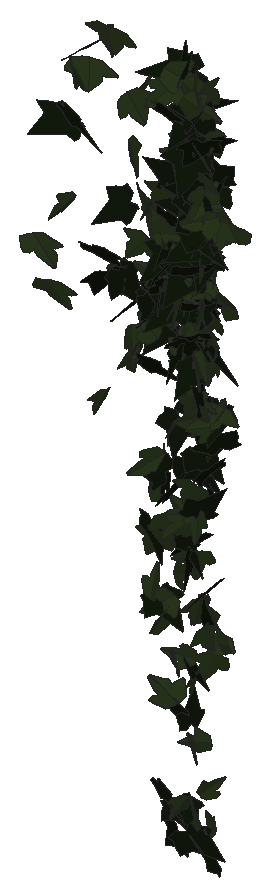
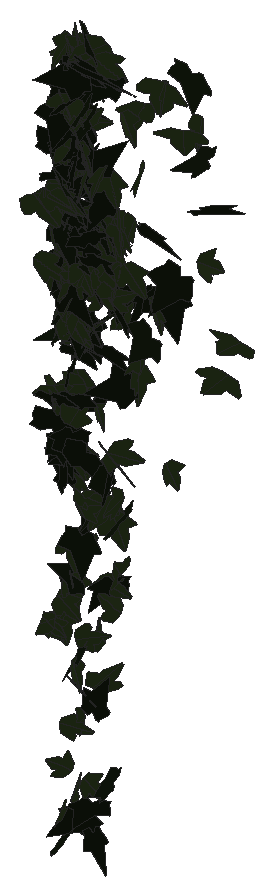
# SketchUp Ruby script. Lengths in millimetres.
U = 1.mm
M = Sketchup.active_model
def pt(a) = Geom::Point3d.new(a.map { |v| v * U })
def face(e, loops, mat)
  f = e.add_face(loops[0].map { |a| pt(a) })
  loops[1..].each { |l| e.add_face(l.map { |a| pt(a) }).erase! }
  f.material = f.back_material = mat if mat
  f
end
# faces: each face lists its corners as indices into pts; further lists are holes
def faces(e, pts, list, mat = nil) = list.each { |f| face(e, (f[0].is_a?(Array) ? f : [f]).map { |l| l.map { |i| pts[i] } }, mat) }
# xy, xz, yz: faces in a plane at the given z, y or x. An outline is a flat list of corners, or four numbers for a rectangle; further outlines are holes
def ring(l) = l.size == 4 ? [[l[0], l[1]], [l[2], l[1]], [l[2], l[3]], [l[0], l[3]]] : l.each_slice(2).to_a
def flat(e, list, mat, &to3) = list.each { |f| face(e, (f[0].is_a?(Array) ? f : [f]).map { |l| ring(l).map { |u, v| to3.(u, v) } }, mat) }
def xy(e, z, list, mat = nil) = flat(e, list, mat) { |x, y| [x, y, z] }
def xz(e, y, list, mat = nil) = flat(e, list, mat) { |x, z| [x, y, z] }
def yz(e, x, list, mat = nil) = flat(e, list, mat) { |y, z| [x, y, z] }
def lines(e, pts, list) = list.each { |a, b| e.add_line(pt(pts[a]), pt(pts[b])) }
# prism: a flat outline (further loops are holes) pulled along v
def prism(e, loops, v, mat = nil)
  f = face(e, loops, mat); d = Geom::Vector3d.new(v.map { |x| x * U })
  f.pushpull(f.normal.samedirection?(d) ? d.length : -d.length)
end
def box(e, o, s, mat = nil) = prism(e, [[o, [o[0] + s[0], o[1], o[2]], [o[0] + s[0], o[1] + s[1], o[2]], [o[0], o[1] + s[1], o[2]]]], [0, 0, s[2]], mat)
def at(x, y, z, deg = 0) = Geom::Transformation.translation(pt([x, y, z])) * Geom::Transformation.rotation(ORIGIN, Z_AXIS, deg.degrees)
def axes(o, x, y, z) = Geom::Transformation.new([*x, 0, *y, 0, *z, 0, *pt(o).to_a, 1])
def part(name) = M.definitions.add(name)
# library, detail: a bought-in or finely detailed component or shape, given as its bounding box
def library(name, o, s) = part(name).tap { |d| box(d.entities, o, s) }
def detail(e, o, s) = box(e.add_group.entities, o, s)
def put(e, d, t, mat = nil) = e.add_instance(d, t).tap { |i| i.material = mat if mat }
def group(e, t, mat = nil) = e.add_group.tap { |g| g.transformation = t; g.material = mat if mat }.entities
root = M.entities
M.materials.add("efeu1").color = [18, 25, 13]
M.materials.add("efeu2").color = [43, 57, 29]
c1 = part("ivyleaf_10")
p = [[0,12.8,-0.8],[-1.5,51.3,-10.9],[-4.9,51,-11.6],[-13.6,26.5,-7.3],[-13.2,15.9,-4.6],[-21.1,19.3,-7.2],
  [-29.5,16.3,-8.3],[-29.2,8.3,-6.2],[-19.7,-9.8,0.5],[-7.6,-13,4],[1,-12.2,5.8],[-0.4,51.1,-11.1],
  [-1.5,51.1,-10.9],[1,-12.4,5.9],[16.9,-12.4,3.5],[35.1,9.1,-5.1],[35,12.9,-6.1],[20.5,16.4,-4.9],
  [15.8,15,-3.8],[15.3,27.6,-7.1],[12.8,31.3,-7.8]]
faces(c1.entities,p,[[0,1,2,3,4,5,6,7,8,9,10],[11,12,0,13,14,15,16,17,18,19,20]],"efeu2")
c2 = part("ivyleaf_9")
p = [[39.1,54.8,31.7],[34.5,51.8,30.2],[-5.3,25.2,17.3],[-17.9,28.3,20.9],[-21.6,21.7,17],[-20.2,4.3,5.3],
  [-22.9,-0.3,2.5],[-17.1,-4,-0.6],[-2,-2.1,-1.2],[-0.7,-15.4,-10.1],[16.6,-22.3,-16.7],[21.1,-15.1,-12.5],
  [32.7,-10.7,-11],[46.1,-1.8,-6.6],[30.8,11.2,3.8]]
faces(c2.entities,p,[[0,1,2,3,4,5,6,7,8,9,10,11,12,13,14]],"efeu1")
put(root,c1,axes([372.2,960.3,1197.6],[1.15006,0.11496,0.41764],[0.78292,0.07226,-0.6151],[-0.25826,0.73099,-0.00488]))
put(root,c1,axes([400,960.9,1128.9],[-1.30327,0.0523,-0.27904],[0.53054,-0.01407,-0.68674],[-0.10229,-0.73932,-0.00667]))
put(root,c2,axes([421.9,977.2,1421.7],[-1.00927,-0.38728,0.42101],[-0.51697,-0.33475,-0.65008],[0.95813,-0.58857,0.09272]))
put(root,c1,axes([448.2,943.8,1302.7],[0.11801,-0.42644,0.64744],[0.10159,-0.64562,-0.43035],[1.47197,0.07874,-0.0222]))
put(root,c1,axes([464.4,937.8,1540.5],[-0.85455,0.60602,0.29472],[-0.46324,0.1844,-0.74999],[-1.19596,-0.50445,0.07991]))
put(root,c1,axes([465.1,971.6,1534.5],[1.29236,0.42585,-0.00571],[-0.00973,-0.00259,-0.80153],[-0.8105,0.67906,0.00052]))
put(root,c1,axes([480.6,988.2,954.1],[-0.03222,-0.68539,0.18089],[0.09045,-0.18163,-0.68375],[1.34607,-0.0042,0.05028]))
put(root,c2,axes([459.3,927.2,1470.8],[0.93119,-0.64159,-0.02055],[-0.02246,0.01684,-0.80686],[1.22148,0.48942,0.00083]))
put(root,c2,axes([499.9,910,1599.1],[0.14786,0.79183,0.24157],[0.07495,0.23882,-0.79549],[-1.5738,0.08577,-0.01519]))
put(root,c1,axes([504.1,977.9,1603.5],[-1.55947,0.07604,0.0471],[-0.09715,-0.04109,-0.82165],[-0.13979,-0.81972,0.04556]))
put(root,c1,axes([506.9,969.1,1599.3],[-0.54473,0.71836,0.28114],[-0.41194,0.21304,-0.7647],[-1.40918,-0.33997,0.11487]))
put(root,c2,axes([511.9,926.8,1248.2],[1.12167,0.31654,-0.15049],[-0.24046,0.11759,-0.9568],[-0.35359,0.92418,0.17328]))
put(root,c2,axes([534.4,928.4,1211.8],[0.14646,0.89185,-0.37066],[-0.14417,-0.35714,-0.8976],[-1.16943,0.15573,0.06423]))
put(root,c1,axes([539.5,952.4,1202.4],[0.3105,-0.74174,0.09498],[0.0709,-0.08903,-0.75928],[1.42145,0.16647,0.01713]))
put(root,c1,axes([541.6,951,1199.4],[0.86184,-0.57711,-0.21937],[-0.1272,0.22463,-0.72892],[1.16813,0.45025,0.08248]))
put(root,c2,axes([555,955.7,1331.1],[-1.07704,0.07844,0.0797],[-0.09649,0.01043,-0.88629],[-0.09645,-0.88635,-0.00338]))
put(root,c2,axes([550.1,948.7,1140.2],[0.36841,0.62954,0.63039],[0.12358,0.63704,-0.6847],[-1.07986,0.28768,0.13671]))
put(root,c1,axes([572.3,975.4,1260],[-0.81055,-0.15305,0.53219],[-0.58352,-0.26031,-0.67196],[0.34047,-0.81048,0.11532]))
put(root,c2,axes([554.8,938.1,1216],[0.26893,-0.55459,-0.74191],[-0.35685,0.68193,-0.59666],[1.07224,0.36604,-0.0125]))
put(root,c1,axes([565.9,986.1,1531],[0.17354,-0.79941,-0.00383],[-0.00164,0.00376,-0.80459],[1.52145,0.09118,-0.00043]))
put(root,c1,axes([561.7,957.9,1428.7],[-0.3786,0.85759,-0.09989],[0.01505,-0.10173,-0.91172],[-1.05322,-0.30973,0.02288]))
put(root,c1,axes([567.5,952.8,1072.9],[-0.05104,-0.86716,-0.26414],[0.04909,0.26238,-0.86776],[1.10483,-0.05172,0.02635]))
put(root,c1,axes([564.9,954.9,1104],[-0.00627,0.90595,-0.20035],[-0.06105,-0.20033,-0.90459],[-1.13032,0.00579,0.04997]))
put(root,c1,axes([568.3,972.8,1342.7],[-0.79907,0.59718,-0.04404],[0.01983,-0.0475,-0.88602],[-0.73027,-0.65473,0.02412]))
put(root,c1,axes([574.7,939,1525.5],[0.52902,0.73756,0.41788],[0.0829,0.43763,-0.84292],[-1.03089,0.41369,0.14666]))
put(root,c1,axes([587.8,977.8,1321.1],[-0.99279,0.32533,-0.09594],[-0.04917,-0.34034,-0.81227],[-0.41087,-0.74537,0.32902]))
put(root,c1,axes([591.6,966.7,1343.1],[0.1882,-0.7562,-0.4352],[-0.11248,0.42535,-0.77176],[1.05848,0.17965,-0.00463]))
put(root,c2,axes([589.3,982,1190.5],[-0.82299,0.10769,-0.48965],[0.59514,-0.04845,-0.68271],[-0.14116,-0.83215,-0.02362]))
put(root,c1,axes([606.9,978.3,1202.4],[0.44164,0.25231,0.76167],[-0.79965,-0.38899,0.44037],[0.56462,-0.74825,0.0279]))
put(root,c1,axes([597.9,969.1,1251.8],[-0.70587,0.56927,0.3834],[-0.3345,0.26799,-0.81168],[-0.76762,-0.64026,0.00114]))
put(root,c2,axes([576.1,966.5,1054.1],[0.96505,-0.14261,0.40968],[0.50414,-0.01149,-0.80187],[0.16101,0.89074,0.05524]))
put(root,c1,axes([602.5,960.3,843.1],[-0.00471,0.0414,0.85618],[-0.36385,0.80263,-0.04016],[-0.98042,-0.29807,0.01079]))
put(root,c2,axes([606.2,989.1,1119.3],[-0.9618,-0.19067,-0.09418],[0.11187,0.02148,-0.81109],[0.23408,-0.79368,0.00067]))
put(root,c2,axes([595.2,959.4,1179.9],[0.5578,-0.66173,-0.24568],[-0.11617,0.24126,-0.72265],[1.33837,0.29673,0.03967]))
put(root,c1,axes([623.9,942.2,911.4],[0.32955,0.36267,-0.81961],[-0.7113,-0.57904,-0.44837],[-0.83046,0.63987,0.05879]))
put(root,c2,axes([620,932.6,1171.3],[-0.28694,-0.4745,0.78731],[0.40185,0.71521,0.52944],[-1.047,0.40454,-0.01257]))
put(root,c2,axes([620.4,965.8,852.7],[-0.02977,-0.46377,0.69519],[0.19297,0.68035,0.45943],[-1.00111,0.14494,0.06788]))
put(root,c1,axes([621.7,932.4,1134.3],[-0.0226,0.82433,0.30778],[-0.00145,-0.30787,0.8245],[1.07349,0.01694,0.00759]))
put(root,c1,axes([635.3,941.4,1382.9],[-0.91558,-0.03693,0.36902],[-0.44798,-0.04282,-0.75105],[0.06345,-0.83519,0.02219]))
put(root,c1,axes([636.5,929.2,785],[-0.93133,-0.24462,0.40341],[-0.46899,-0.12232,-0.80162],[0.33366,-0.85471,-0.00073]))
put(root,c2,axes([635.9,989.6,1266.4],[-0.94207,-0.18682,0.08903],[-0.10462,-0.02414,-0.79446],[0.22978,-0.77693,0.00328]))
put(root,c1,axes([629.6,969.6,1233.1],[-0.25102,-0.74677,0.15508],[0.07612,-0.16394,-0.7554],[1.44957,-0.12071,0.06652]))
put(root,c1,axes([612.1,981.4,1245.3],[0.8025,-0.11396,0.55782],[0.66531,-0.11876,-0.66733],[0.19955,0.85425,-0.01835]))
put(root,c2,axes([637.8,930.6,1211.6],[0.09032,-0.04347,-0.87338],[-0.93526,0.41847,-0.08581],[0.51327,0.77017,-0.00268]))
put(root,c2,axes([645.6,930.8,898],[-0.63228,0.53164,0.3765],[-0.31485,0.27419,-0.74243],[-0.72975,-0.57893,-0.00588]))
put(root,c2,axes([634.3,909.4,1177.6],[0.08799,0.76052,0.31916],[-0.00297,0.32058,-0.76333],[-1.00622,0.06556,0.03016]))
put(root,c1,axes([630.5,918.9,690.7],[0.03169,0.62244,-0.59236],[0.03568,0.59165,0.62297],[1.04769,-0.03898,-0.0033]))
put(root,c1,axes([638.7,925.8,1243.9],[-0.91204,0.28675,0.34177],[-0.39479,0.11056,-0.8006],[-0.37467,-0.81452,0.01165]))
put(root,c2,axes([616.3,940.6,791.5],[0.27256,-0.82251,0.41936],[0.14402,-0.40247,-0.85228],[1.11712,0.25257,0.00756]))
put(root,c2,axes([644.8,965.8,250.5],[0.3792,0.09051,-0.77293],[-0.93543,-0.10668,-0.32083],[-0.16232,0.82622,0.04324]))
put(root,c1,axes([644.9,930.9,1302.7],[-0.71315,0.37335,0.53244],[-0.57766,0.24638,-0.6926],[-0.54381,-0.75133,0.03746]))
put(root,c2,axes([662.2,984,1587.1],[-1.4231,0.19425,0.27152],[-0.56243,-0.07525,-0.75999],[-0.29561,-0.79195,0.13881]))
put(root,c1,axes([634.1,963.4,1404.5],[-0.20146,0.84579,0.30778],[-0.11504,0.29494,-0.86109],[-1.09202,-0.18711,0.03393]))
put(root,c1,axes([648.2,936,675.7],[0.56187,0.2555,-0.64393],[-0.71255,-0.27265,-0.52591],[-0.45454,0.74325,0.02844]))
put(root,c1,axes([637.9,924.3,626.2],[0.18448,-0.72012,0.44867],[-0.02525,0.45248,0.73319],[-1.03481,-0.13942,0.06209]))
put(root,c2,axes([639.4,942.1,1216.2],[-0.3046,0.76452,-0.27388],[-0.10764,0.2593,0.80425],[0.98489,0.26478,0.00319]))
put(root,c2,axes([628.2,943.2,336.5],[0.71988,-0.6358,0.02525],[0.02851,-0.01276,-0.86738],[0.77576,0.59047,0.00845]))
put(root,c2,axes([655.5,959.2,1404.2],[0.2011,0.03859,0.90855],[-1.06372,-0.2556,0.16904],[0.31517,-0.8873,-0.00918]))
put(root,c2,axes([648.3,962.2,464.6],[0.61026,-0.44274,0.48734],[-0.35901,0.39717,0.66287],[-0.71858,-0.57443,0.0827]))
put(root,c2,axes([636.3,933.7,679.7],[0.04196,-0.62455,-0.66184],[-0.05115,0.66052,-0.62549],[1.10902,0.05409,-0.00381]))
put(root,c1,axes([652.1,942.7,500.6],[0.44862,0.64982,0.52167],[-0.32248,-0.4498,0.74662],[0.96414,-0.45281,0.00699]))
put(root,c2,axes([651.5,933,1302.8],[-0.8664,0.39382,-0.48971],[0.51156,-0.25346,-0.8119],[-0.57105,-0.82457,0.01567]))
put(root,c1,axes([657.6,934.8,1578],[0.77414,0.32422,-0.62424],[-0.70321,-0.2422,-0.71171],[-0.49188,0.85654,0.03504]))
put(root,c2,axes([641.1,920.9,1230],[0.63456,0.51175,0.34844],[0.30844,0.23985,-0.72965],[-0.68947,0.57829,-0.00572]))
put(root,c2,axes([656.7,945.1,1282.3],[-0.99369,-0.43484,0.17482],[-0.06122,-0.2676,-0.8994],[0.56848,-0.7889,0.20872]))
put(root,c2,axes([645.2,939,1349.1],[0.9734,0.04653,-0.34518],[-0.41976,-0.02892,-0.79918],[-0.0661,0.86885,-0.00812]))
put(root,c1,axes([662.4,976.8,1233.3],[-0.78347,-0.09933,0.44384],[-0.53824,-0.05057,-0.64967],[0.13484,-0.779,-0.01442]))
put(root,c2,axes([660.2,923.2,1270.5],[-0.51021,0.7609,-0.37313],[0.19251,-0.3389,-0.86795],[-1.01583,-0.4464,0.02292]))
put(root,c1,axes([648,938.3,817.3],[-0.65103,-0.67493,-0.35639],[0.35687,0.22081,-0.85615],[0.86007,-0.60251,0.08547]))
put(root,c1,axes([647.5,946.8,1240.6],[1.00797,0.16039,-0.09412],[0.11089,0.02566,0.84159],[0.19794,-0.83115,0.00782]))
put(root,c2,axes([643.7,936.4,851],[0.21152,0.84027,0.25704],[-0.10999,-0.2436,0.85715],[1.06636,-0.1918,0.03743]))
put(root,c2,axes([672.2,960.9,1580.4],[-0.89934,0.29395,0.34517],[-0.40689,0.0947,-0.79294],[-0.37466,-0.80844,0.03261]))
put(root,c2,axes([669.8,945,1207.5],[-0.20009,0.14057,-0.81785],[-0.98753,0.15657,0.18924],[0.22305,0.81931,0.10416]))
put(root,c2,axes([664.2,961.9,1464.3],[0.46914,0.0148,-0.82165],[-1.00219,0.03215,-0.38388],[0.02788,0.90661,0.02703]))
put(root,c1,axes([637.4,933,1314.1],[-0.16247,-0.10252,0.8129],[0.77775,0.50439,0.16805],[-0.62793,0.65126,-0.00218]))
put(root,c1,axes([668.6,961.6,810.5],[0.61348,0.01488,0.69028],[-0.84233,0.0057,0.50284],[0.00507,-0.854,0.01539]))
put(root,c2,axes([655.3,981.4,1293.2],[-0.58519,-0.73241,0.04364],[-0.04061,-0.03036,-0.87543],[0.8942,-0.48069,-0.0112]))
put(root,c1,axes([656.5,939.4,1171.2],[0.22888,-0.54419,0.68042],[-0.24742,0.64962,0.57548],[-1.03375,-0.27596,0.01291]))
put(root,c1,axes([657.2,942.7,983.8],[0.32753,-0.76288,0.01785],[0.0073,-0.01682,-0.80874],[0.93094,0.26853,0.00006]))
put(root,c1,axes([668.6,967,1432],[0.35569,-0.21377,-0.73495],[-0.56224,0.5789,-0.3512],[0.74556,0.53854,0.08578]))
put(root,c2,axes([667,937.2,1202.1],[-1.04196,-0.30228,0.06457],[-0.0618,-0.05028,-0.90547],[0.37201,-0.85502,0.03042]))
put(root,c2,axes([663.8,972,763.5],[0.13353,0.89281,-0.02684],[-0.00417,-0.02662,-0.89949],[-1.08971,0.1095,0.00016]))
put(root,c1,axes([659.2,950.6,1109],[0.13121,0.60025,-0.47323],[0.01532,0.47644,0.60717],[0.93239,-0.0923,0.05662]))
put(root,c2,axes([649.1,966.9,303.9],[-0.17094,-0.56673,-0.59091],[0.18281,0.57163,-0.58376],[0.98201,-0.20507,0.00581]))
put(root,c1,axes([661.8,965.3,1394.9],[-0.51962,0.65941,0.36634],[-0.22015,0.31942,-0.78476],[-0.89357,-0.46215,-0.01968]))
put(root,c2,axes([646.5,917.6,1547.9],[1.20569,-0.04104,-0.0708],[-0.08398,0.04707,-0.98814],[0.05399,0.98969,0.04406]))
put(root,c1,axes([677.7,956.6,1461.2],[0.04398,0.11079,0.8386],[-0.94914,0.33385,-0.01066],[-0.40513,-0.77013,0.11602]))
put(root,c1,axes([656.8,979.7,1205.7],[-0.03724,-0.0414,0.8464],[0.38478,-0.78666,-0.0271],[0.95957,0.31384,0.04371]))
put(root,c1,axes([677.3,952.8,576.7],[-0.14843,-0.06904,-0.71395],[-0.82512,-0.23015,0.13751],[-0.29147,0.6867,-0.0257]))
put(root,c2,axes([680.2,959.9,1444.9],[-0.39112,0.10626,-0.83579],[-0.96942,0.25911,0.33774],[0.34166,0.85684,0.00152]))
put(root,c2,axes([662,945.6,1117.9],[-0.6446,0.10109,-0.57915],[0.66354,-0.21159,-0.53312],[-0.27232,-0.75486,0.07187]))
put(root,c2,axes([678.9,964,1361.2],[-0.39668,-0.07178,0.756],[-0.81788,-0.3592,-0.32243],[0.43522,-0.74043,0.08313]))
put(root,c1,axes([665.1,935.8,563.2],[-0.692,0.43189,0.2144],[0.19254,-0.14651,0.71264],[0.55585,0.58842,0.02007]))
put(root,c1,axes([680.5,981.9,1134.7],[-0.65914,-0.30081,0.60182],[-0.60004,-0.3501,-0.61653],[0.56011,-0.72906,0.04775]))
put(root,c2,axes([661.3,948.1,989.6],[-0.23414,-0.79272,0.06221],[-0.01092,-0.06184,-0.8156],[0.97003,-0.19204,0.00583]))
put(root,c1,axes([676.1,944.8,813.1],[-0.3735,-0.41951,0.59721],[-0.36745,-0.51728,-0.51776],[0.81103,-0.42756,0.04045]))
put(root,c2,axes([675.5,955.1,1126.2],[0.14636,0.66516,-0.5349],[-0.2,-0.51214,-0.67363],[-1.02195,0.19549,0.05523]))
put(root,c2,axes([684,954.2,1251],[-0.07573,0.04842,0.85915],[-0.61977,0.6932,-0.07578],[-0.84736,-0.51134,-0.02136]))
put(root,c2,axes([676.1,936.8,1603.8],[0.08519,0.26703,0.89686],[-0.10209,0.89753,-0.26072],[-1.13706,-0.06057,0.09061]))
put(root,c2,axes([681.8,982.4,1185.5],[0.17676,0.20474,-0.75608],[-0.75084,-0.4459,-0.23868],[-0.59117,0.62755,0.07708]))
put(root,c1,axes([673.8,930.3,731.9],[-0.22426,0.33024,0.71417],[-0.40934,0.63048,-0.3779],[-0.86828,-0.38253,-0.0063]))
put(root,c1,axes([672.5,946.6,324.3],[-0.11601,-0.58735,0.38305],[-0.06945,-0.37882,-0.59499],[0.85267,-0.11077,0.00366]))
put(root,c1,axes([683.9,958.8,1468.8],[-0.60153,-0.19256,-0.65801],[-0.69605,-0.33422,0.52531],[-0.46384,0.75125,0.06504]))
put(root,c1,axes([677.8,977,968.7],[-0.48715,-0.47547,-0.48066],[-0.37912,-0.3667,0.6209],[-0.73255,0.50597,-0.0017]))
put(root,c1,axes([672.1,976.4,1133.3],[0.95999,-0.39093,-0.10725],[-0.09956,0.07663,-0.87805],[0.48444,0.79045,0.03208]))
put(root,c1,axes([670.7,944.2,1195.9],[0.07838,0.55084,-0.5505],[-0.10248,-0.54424,-0.55439],[-0.94455,0.10476,0.01447]))
put(root,c1,axes([675.4,974.1,535.3],[0.24056,-0.7557,0.00758],[0.01215,-0.00523,-0.78095],[0.92192,0.19726,0.00832]))
put(root,c2,axes([680.1,956,1137.3],[0.44708,0.77889,-0.21045],[-0.27503,-0.12309,-0.84811],[-0.94512,0.40427,0.14724]))
put(root,c2,axes([667.7,963.6,565.3],[0.71436,-0.44412,-0.42017],[-0.40128,0.26158,-0.73487],[0.62873,0.67155,0.00837]))
put(root,c1,axes([660,935.3,1603.1],[0.39775,0.37985,0.79426],[0.57872,0.63773,-0.49971],[-0.90487,0.57484,0.02954]))
put(root,c1,axes([680.6,966.5,748.8],[-0.8673,-0.56861,0.02747],[-0.02589,-0.01744,-0.91032],[0.69402,-0.71121,0.00037]))
put(root,c1,axes([676.7,949.7,1382.8],[0.4421,-0.84765,0.07309],[0.04131,-0.06501,-0.92184],[1.03714,0.36391,0.00557]))
put(root,c2,axes([663.7,958.6,783.8],[0.50846,-0.82191,-0.03889],[-0.04152,0.02634,-0.92135],[1.00299,0.41775,-0.01843]))
put(root,c2,axes([672.9,982,1010],[-0.56067,-0.51143,-0.38377],[0.30945,0.28801,-0.68757],[0.71607,-0.52491,-0.00335]))
put(root,c1,axes([692.6,944.3,1459.5],[0.17441,0.23367,0.83932],[-0.73292,-0.58956,0.26646],[0.76981,-0.61425,0.06353]))
put(root,c2,axes([682.8,966.4,1085.2],[-0.93899,-0.37313,-0.11884],[0.14713,0.02348,-0.85478],[0.45453,-0.77843,0.03118]))
put(root,c1,axes([668.8,965.3,1207.1],[0.38258,0.53986,0.63798],[0.31402,0.5859,-0.62231],[-0.97004,0.40259,0.05016]))
put(root,c2,axes([662.7,958,1482.5],[0.80487,-0.63387,0.08771],[0.077,-0.06091,-0.9149],[0.77689,0.66274,-0.00019]))
put(root,c2,axes([661.9,966.9,910.6],[-0.07184,-0.17184,-0.88111],[0.797,0.59743,-0.16017],[0.75118,-0.65031,0.08568]))
put(root,c2,axes([688,970.8,1388.1],[0.12069,-0.36904,0.7982],[-0.1001,0.79585,0.37813],[-1.06816,-0.11628,0.05475]))
put(root,c1,axes([688.1,965.9,993.6],[-0.06293,-0.05444,-0.84053],[-0.5143,-0.72738,0.07298],[-0.88963,0.42435,0.01726]))
put(root,c1,axes([694.7,969.6,425.1],[-0.08415,-0.06168,0.68232],[-0.62827,-0.44761,-0.09252],[0.55125,-0.51957,-0.0013]))
put(root,c1,axes([692.6,982.4,647],[-0.51619,-0.28697,0.47653],[-0.4661,-0.28524,-0.511],[0.49326,-0.56985,0.01581]))
put(root,c1,axes([691.8,948.9,1022.9],[-0.96038,0.03037,0.34186],[-0.41798,-0.01905,-0.78722],[-0.02471,-0.85801,0.02958]))
put(root,c1,axes([697.6,968.5,1208.4],[-0.58532,-0.03468,0.59494],[-0.72186,-0.0634,-0.48085],[0.08675,-0.76165,0.01294]))
put(root,c2,axes([671.2,967,1491.6],[0.11272,-0.56269,0.59128],[0.15847,-0.57733,-0.56972],[0.98311,0.15758,0.02404]))
put(root,c2,axes([692,945.5,1384.6],[-0.40351,-0.73089,0.28254],[0.13911,0.25853,0.80224],[-0.94582,0.34984,-0.00255]))
put(root,c2,axes([691.6,940.1,472.9],[-0.79045,0.38477,-0.14043],[-0.16194,0.05138,0.75319],[0.47274,0.66096,0.0232]))
put(root,c2,axes([701.3,967.4,1365.7],[-0.76215,0.63506,0.01941],[-0.01753,0.01309,-0.89083],[-0.77494,-0.62488,0.00106]))
put(root,c2,axes([678.4,955.3,1344.6],[0.53715,-0.50963,-0.6154],[0.50846,-0.45301,0.67333],[-0.8317,-0.60609,0.01419]))
put(root,c1,axes([690.5,961.3,673.1],[-0.2272,-0.83777,0.00724],[-0.00156,-0.00714,-0.85822],[1.02212,-0.18623,0.0003]))
put(root,c2,axes([694.6,935,1268.3],[-1.02644,-0.44479,-0.05657],[0.07142,0.01028,-0.95151],[0.54233,-0.84318,0.01824]))
put(root,c1,axes([682,949.9,433.5],[-0.45315,0.46703,-0.38856],[0.28169,-0.31274,-0.59661],[-0.68558,-0.43719,0.01169]))
put(root,c1,axes([674.2,968.1,1025.7],[-0.44838,0.06462,-0.64624],[0.77536,-0.11715,-0.37315],[-0.16319,-0.73415,0.00266]))
put(root,c1,axes([685.1,982.6,1151.2],[-0.2688,0.35121,0.67401],[0.3409,-0.61518,0.41189],[0.86229,0.35269,0.04727]))
put(root,c1,axes([699.4,938.6,885.8],[-0.87668,-0.22796,0.34437],[-0.40313,-0.0972,-0.75386],[0.30223,-0.7909,-0.00661]))
put(root,c1,axes([688.9,955.2,1097],[-0.63983,0.67905,-0.13617],[-0.00135,-0.17162,-0.85161],[-0.84494,-0.51394,0.10447]))
put(root,c1,axes([704.4,980.9,1344.8],[0.52804,0.00626,-0.70011],[-0.85404,-0.00997,-0.43287],[-0.01436,0.82303,0.00008]))
put(root,c1,axes([679,981.7,1153.6],[-0.674,0.36477,-0.55973],[0.58418,-0.29033,-0.66182],[-0.56842,-0.73091,-0.01646]))
put(root,c2,axes([676.8,952,265.6],[-0.057,-0.17198,-0.85274],[0.4061,0.78544,-0.17665],[0.98051,-0.3353,0.02359]))
put(root,c2,axes([709,941.4,1408.7],[-0.3163,0.53962,0.66936],[-0.48909,0.5426,-0.59271],[-0.92792,-0.46993,0.08425]))
put(root,c1,axes([695.5,966.4,1429.7],[0.43649,0.60825,-0.53666],[-0.40491,-0.42542,-0.70344],[-0.90297,0.48479,0.05602]))
put(root,c2,axes([698.7,936.5,1547.4],[-1.12504,-0.12921,-0.2486],[0.30403,0.01254,-0.93092],[0.15621,-0.955,0.02141]))
put(root,c1,axes([696.3,949.4,294.8],[-0.51643,0.60693,0.02947],[0.01196,-0.02909,0.73991],[0.74123,0.42333,0.00859]))
put(root,c2,axes([686.3,966.8,934.7],[-0.03498,-0.48102,-0.68461],[0.06038,0.68284,-0.48185],[1.01899,-0.05697,0.00505]))
put(root,c2,axes([687.5,942.2,761.5],[-0.11842,0.09646,-0.77419],[0.77907,-0.43838,-0.13469],[-0.54682,-0.64546,-0.02422]))
put(root,c2,axes([689.5,949.8,675.5],[-0.10244,0.74638,-0.18721],[-0.02589,0.186,0.75109],[0.93843,0.0866,0.00029]))
put(root,c1,axes([698.9,982.8,266],[-0.24435,0.62397,0.045],[0.01055,-0.04448,0.65531],[0.76315,0.2004,0.00535]))
put(root,c2,axes([698,939.6,1472.5],[-0.82394,-0.65984,-0.16469],[0.12195,0.13328,-0.94386],[0.82069,-0.68226,-0.0251]))
put(root,c1,axes([690.6,955.5,1209.4],[0.69344,-0.61409,0.30724],[0.40659,-0.22918,-0.7114],[1.242,0.41789,0.06135]))
put(root,c2,axes([697.5,960.9,1021.6],[-0.18165,0.32286,0.77607],[-0.32734,-0.76517,0.26685],[0.97182,-0.19739,0.23495]))
put(root,c2,axes([687,988.6,857.7],[0.04589,-0.06093,0.8045],[0.16866,-0.79298,-0.06652],[0.96974,0.1408,-0.0265]))
put(root,c2,axes([702.8,985.4,214.5],[0.18646,-0.7994,0.07284],[0.00168,0.07441,0.81373],[-0.9793,-0.15207,0.01526]))
put(root,c1,axes([715.5,983.2,1349.4],[-0.47123,-0.16286,0.72061],[-0.79034,-0.31623,-0.41871],[0.43327,-0.75397,0.01996]))
put(root,c2,axes([714.1,946.2,1319.2],[-1.0678,-0.15672,0.29435],[-0.34115,-0.10553,-0.88766],[0.22167,-0.91737,0.05183]))
put(root,c2,axes([721.5,926.9,1416.7],[-0.29296,0.10546,-0.90134],[-1.00754,-0.41188,0.17183],[-0.45893,0.83692,0.19814]))
put(root,c2,axes([688.1,948.4,1550.2],[0.10727,0.50047,-0.73814],[0.1162,0.7322,0.50779],[1.08178,-0.12828,0.01865]))
put(root,c1,axes([704.4,972.5,980.7],[-0.1402,0.23357,0.79351],[-0.08538,-0.80101,0.22564],[1.00553,-0.03545,0.1298]))
put(root,c2,axes([712.6,981.5,944.5],[0.55516,0.13697,0.71958],[-1.271,-0.2685,0.32182],[0.57278,-0.72856,0.01668]))
put(root,c1,axes([717.5,921,1599.3],[-0.32981,0.34773,0.74608],[-0.79605,0.3882,-0.41736],[-0.6122,-0.69212,0.14075]))
put(root,c1,axes([700.2,959.3,1502.3],[-0.90526,-0.33576,-0.3258],[0.37324,0.11391,-0.81419],[0.43182,-0.80235,0.02074]))
put(root,c2,axes([711.6,961.8,913.2],[-0.14151,0.7771,-0.22786],[0.0709,-0.22161,-0.78535],[-0.98543,-0.12753,-0.02378]))
put(root,c2,axes([686.5,927.8,1260.4],[0.84035,0.54607,-0.17039],[0.15592,0.11305,0.87896],[0.68024,-0.70051,0.00902]))
put(root,c2,axes([696.2,965.6,1505.6],[0.02859,-0.83752,-0.09939],[-0.00691,0.09927,-0.83785],[1.02892,0.02394,-0.00286]))
put(root,c2,axes([706.8,988.4,1392.7],[-0.5607,-0.64323,0.16682],[-0.12148,-0.13388,-0.79054],[0.80154,-0.47025,-0.00312]))
put(root,c1,axes([707.8,977,1008.3],[1.17079,0.37241,-0.28496],[-0.46271,-0.14865,-0.71911],[-0.76314,0.66147,-0.00117]))
put(root,c1,axes([698,945.8,1401.2],[-0.62855,0.4824,-0.55928],[0.35202,-0.49625,-0.69384],[-0.82946,-0.57616,0.12935]))
put(root,c2,axes([713.5,971.4,1420.7],[0.65837,-0.04797,0.72193],[-0.83125,0.26928,0.52721],[-0.29694,-0.86017,0.12479]))
put(root,c1,axes([690.5,939.7,1588.4],[-0.60361,0.10545,-0.74982],[0.85837,-0.26703,-0.5018],[-0.34143,-0.85774,0.06404]))
put(root,c2,axes([706,992.7,1005.2],[-0.80687,-0.42226,-0.29014],[0.36076,0.07228,-0.77925],[0.51043,-0.71858,0.09211]))
put(root,c2,axes([716.9,949.6,1273.9],[-0.18641,0.91899,-0.03563],[0.0015,-0.03592,-0.93159],[-1.12201,-0.15273,0.00467]))
put(root,c1,axes([723.6,982.4,601.4],[-0.18904,-0.02959,0.67515],[-0.82308,-0.03346,-0.1563],[0.04789,-0.69189,-0.02131]))
put(root,c2,axes([708.9,963,1487],[0.49972,0.72474,-0.05077],[-0.03233,-0.04333,-0.83248],[-0.88576,0.41046,0.00175]))
put(root,c1,axes([712.1,963.3,1199.9],[0.25615,-0.61433,-0.45784],[-0.02094,0.46325,-0.62483],[1.45803,0.11458,0.07146]))
put(root,c2,axes([731.5,928.7,1561.1],[-0.32064,-0.0857,-0.87804],[-0.9995,-0.31617,0.27609],[-0.39928,0.86027,0.01399]))
put(root,c1,axes([704.2,960.7,344.3],[-0.11243,-0.40307,0.54853],[0.13987,0.53643,0.41345],[-0.81858,0.14702,-0.00469]))
put(root,c1,axes([713.5,960.5,1356.9],[-0.65609,-0.74544,-0.00437],[0.00181,0.00432,-0.91918],[0.90945,-0.53778,-0.00132]))
put(root,c2,axes([691.8,966.2,661.2],[0.45331,-0.36728,-0.67008],[0.89591,-0.03437,0.42604],[-0.25774,-0.76543,0.3024]))
put(root,c2,axes([692.6,975.1,1118.7],[0.82127,-0.617,-0.10754],[-0.07306,0.10429,-0.7524],[1.18973,0.43232,0.02803]))
put(root,c1,axes([712.8,986.7,601.9],[0.5703,0.42898,-0.34585],[-0.32209,-0.22373,-0.63435],[-0.59008,0.53672,0.012]))
put(root,c1,axes([724.7,951.7,1189.4],[-0.77397,0.11559,0.54828],[-0.65788,0.09913,-0.64485],[-0.18578,-0.83262,-0.00066]))
put(root,c2,axes([693.2,949,1478.6],[0.35854,-0.53712,0.65414],[0.36085,-0.58363,-0.6121],[0.96752,0.41672,-0.01412]))
put(root,c1,axes([700.4,959.2,1106.3],[0.82849,-0.21797,0.37866],[0.46539,-0.0454,-0.71026],[0.25988,0.77619,0.06479]))
put(root,c2,axes([706.2,931.4,1215.3],[0.83639,0.54044,0.04093],[0.03687,0.02777,-0.87296],[-0.6602,0.68622,0.0031]))
put(root,c1,axes([705.4,935.8,840.7],[0.90219,-0.2878,0.21417],[0.24843,-0.06723,-0.79346],[0.36033,0.76695,0.01082]))
put(root,c2,axes([695.6,939.1,1336.8],[0.5228,-0.63124,-0.41049],[-0.03785,0.43071,-0.67566],[1.43256,0.24175,0.13195]))
put(root,c1,axes([727.7,939.4,1367.6],[0.31661,0.09658,-0.82508],[-0.91491,-0.34459,-0.27621],[-0.43595,0.79332,-0.01953]))
put(root,c1,axes([720.2,945.1,1231.6],[0.06207,0.61239,0.52206],[-0.2625,-0.4937,0.60009],[0.946,-0.17717,0.13227]))
put(root,c1,axes([713.4,947.8,636.4],[-0.16878,-0.78084,-0.30632],[0.2417,0.27125,-0.78094],[0.99436,-0.19848,0.13783]))
put(root,c2,axes([727.2,931.3,1333.5],[-0.48992,0.76426,-0.05938],[0.0121,-0.06185,-0.86311],[-0.93513,-0.4012,0.01994]))
put(root,c2,axes([724.6,924.3,1506.5],[0.13413,0.6776,-0.55936],[-0.17943,-0.54157,-0.68497],[-1.05683,0.17795,0.0453]))
put(root,c1,axes([702.7,960.8,1487.2],[0.01368,-0.17778,-0.85341],[0.57354,-0.7175,0.15564],[-0.8956,-0.4622,0.08664]))
put(root,c2,axes([715.6,952,1297.8],[-0.847,-0.34169,-0.37691],[0.47248,0.05853,-0.76642],[0.40247,-0.78781,0.10653]))
put(root,c1,axes([722.1,979.3,1016],[0.26828,-0.64935,-0.25041],[-0.11704,0.24288,-0.66443],[1.31938,0.15358,-0.00802]))
put(root,c2,axes([709,967.5,1377.8],[-0.10926,0.66133,0.61469],[0.05815,-0.61338,0.66686],[1.09998,0.09812,0.0258]))
put(root,c2,axes([705.4,935,843.9],[-0.09405,-0.2401,0.78728],[0.94504,0.24615,0.15092],[-0.33946,0.75178,0.20203]))
put(root,c2,axes([723.8,911.3,1552.6],[0.14182,0.35827,0.78626],[0.04804,0.79033,-0.36594],[-1.05304,0.08431,0.0892]))
put(root,c2,axes([735.4,929.5,1211.7],[-0.76072,0.46457,0.21404],[-0.22069,0.1154,-0.77743],[-0.58371,-0.64907,0.01498]))
put(root,c1,axes([713.7,938.4,1302.2],[-0.17754,0.52565,-0.67132],[0.19909,-0.65126,-0.54532],[-1.02097,-0.2184,0.0104]))
put(root,c1,axes([735.9,987.2,1330.5],[-1.12282,-0.36304,0.39935],[-0.49796,-0.32507,-0.68206],[0.89838,-0.63393,0.12106]))
put(root,c1,axes([729.1,949.6,591.6],[-0.74612,-0.49514,0.26653],[-0.23155,-0.18893,-0.78646],[0.64577,-0.63982,0.02596]))
put(root,c1,axes([740.3,926.7,1428],[0.09991,-0.01313,-0.8836],[-0.93716,0.43763,-0.0777],[0.53298,0.77197,0.02902]))
put(root,c1,axes([723.2,935.5,1588.5],[0.02068,0.52,0.68475],[-0.23537,0.66972,-0.50381],[-1.02223,-0.14369,0.12985]))
put(root,c1,axes([726.9,929.8,1588.6],[0.55494,-0.71845,-0.31869],[-0.20841,0.26903,-0.85034],[0.93595,0.48589,-0.00039]))
put(root,c1,axes([719.6,943.1,1210.7],[0.02341,0.4415,-0.73467],[-0.04349,-0.7338,-0.44191],[-1.04478,0.04044,0.00194]))
put(root,c1,axes([717,969.6,1108.4],[-0.09982,0.24007,-0.78209],[0.16543,-0.77114,-0.2509],[-0.98428,-0.15396,0.03714]))
put(root,c1,axes([746.1,963.8,1210],[0.2101,0.09635,-0.77376],[-1.10121,0.53397,-0.01606],[0.99477,0.57076,0.14564]))
put(root,c1,axes([719.6,968.9,1337.4],[1.07328,0.10692,0.00564],[0.0065,0.00285,-0.88621],[-0.13046,0.87975,0.00218]))
put(root,c1,axes([729,921.1,1211.8],[-0.51086,0.55679,0.42577],[-0.32585,0.3318,-0.69657],[-0.79061,-0.49652,0.01197]))
put(root,c1,axes([706.2,921.9,1574.5],[-0.53136,-0.01015,-0.81873],[0.99659,-0.06876,-0.4337],[-0.06827,-0.92481,0.04123]))
put(root,c1,axes([729.3,932.2,1412.9],[0.35637,0.58127,-0.60954],[-0.4496,-0.49192,-0.64572],[-0.92399,0.46355,0.07911]))
put(root,c1,axes([717.3,974.7,1280.5],[0.37335,-0.59104,0.59331],[0.45309,-0.47039,-0.66015],[0.91574,0.4737,0.08474]))
put(root,c1,axes([726.1,931.1,1414.2],[0.42219,0.64987,-0.48786],[-0.27683,-0.43189,-0.73627],[-0.95196,0.41381,-0.00226]))
